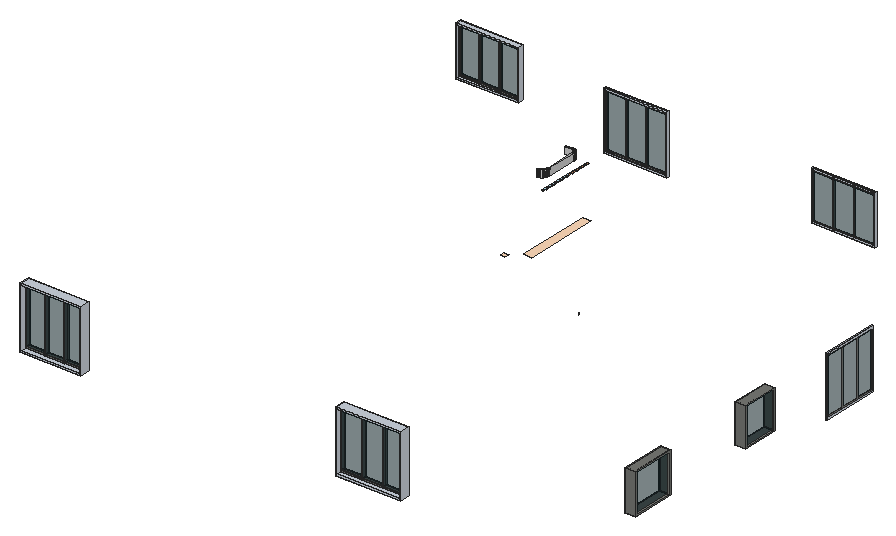
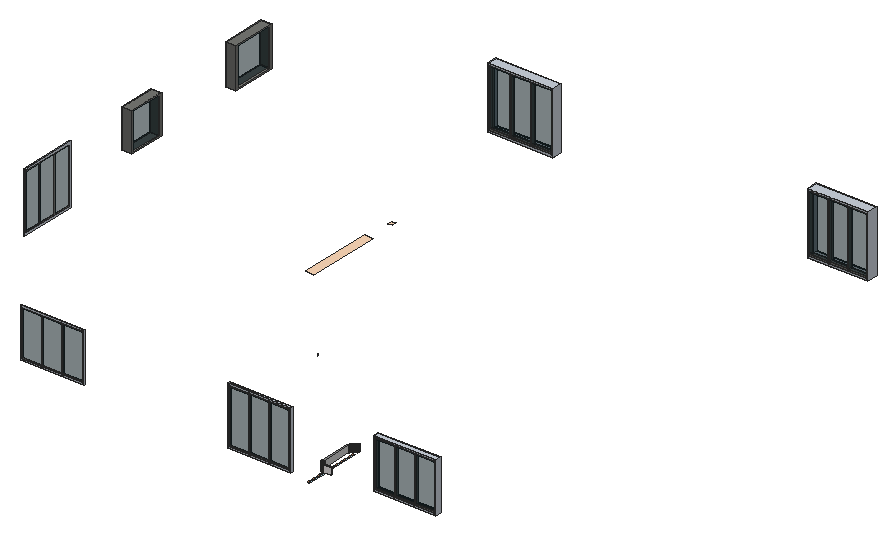
# SketchUp Ruby script. Lengths in inches.
U = 1.inch
M = Sketchup.active_model
def pt(a) = Geom::Point3d.new(a.map { |v| v * U })
def face(e, loops, mat)
  f = e.add_face(loops[0].map { |a| pt(a) })
  loops[1..].each { |l| e.add_face(l.map { |a| pt(a) }).erase! }
  f.material = f.back_material = mat if mat
  f
end
# faces: each face lists its corners as indices into pts; further lists are holes
def faces(e, pts, list, mat = nil) = list.each { |f| face(e, (f[0].is_a?(Array) ? f : [f]).map { |l| l.map { |i| pts[i] } }, mat) }
# xy, xz, yz: faces in a plane at the given z, y or x. An outline is a flat list of corners, or four numbers for a rectangle; further outlines are holes
def ring(l) = l.size == 4 ? [[l[0], l[1]], [l[2], l[1]], [l[2], l[3]], [l[0], l[3]]] : l.each_slice(2).to_a
def flat(e, list, mat, &to3) = list.each { |f| face(e, (f[0].is_a?(Array) ? f : [f]).map { |l| ring(l).map { |u, v| to3.(u, v) } }, mat) }
def xy(e, z, list, mat = nil) = flat(e, list, mat) { |x, y| [x, y, z] }
def xz(e, y, list, mat = nil) = flat(e, list, mat) { |x, z| [x, y, z] }
def yz(e, x, list, mat = nil) = flat(e, list, mat) { |y, z| [x, y, z] }
def lines(e, pts, list) = list.each { |a, b| e.add_line(pt(pts[a]), pt(pts[b])) }
# prism: a flat outline (further loops are holes) pulled along v
def prism(e, loops, v, mat = nil)
  f = face(e, loops, mat); d = Geom::Vector3d.new(v.map { |x| x * U })
  f.pushpull(f.normal.samedirection?(d) ? d.length : -d.length)
end
def box(e, o, s, mat = nil) = prism(e, [[o, [o[0] + s[0], o[1], o[2]], [o[0] + s[0], o[1] + s[1], o[2]], [o[0], o[1] + s[1], o[2]]]], [0, 0, s[2]], mat)
def at(x, y, z, deg = 0) = Geom::Transformation.translation(pt([x, y, z])) * Geom::Transformation.rotation(ORIGIN, Z_AXIS, deg.degrees)
def axes(o, x, y, z) = Geom::Transformation.new([*x, 0, *y, 0, *z, 0, *pt(o).to_a, 1])
def part(name) = M.definitions.add(name)
# library, detail: a bought-in or finely detailed component or shape, given as its bounding box
def library(name, o, s) = part(name).tap { |d| box(d.entities, o, s) }
def detail(e, o, s) = box(e.add_group.entities, o, s)
def put(e, d, t, mat = nil) = e.add_instance(d, t).tap { |i| i.material = mat if mat }
def group(e, t, mat = nil) = e.add_group.tap { |g| g.transformation = t; g.material = mat if mat }.entities
root = M.entities
M.materials.add("Material \#1").color = [140, 140, 140]
M.materials.add("[0006_Pink]").color = [255, 192, 203]
M.materials.add("[0010_Snow]").color = [255, 250, 250]
M.materials.add("[0027_PeachPuff]").color = [255, 218, 185]
M.materials.add("[0095_LightBlue]").color = [173, 216, 230]
M.materials.add("[Carrera Marble]").color = [207, 207, 207]
M.materials.add("[Metal Aluminum Anodized]").color = [202, 209, 219]
M.materials.add("[Metal Seamed]").color = [118, 119, 115]
M.materials.add("[Translucent Glass Tinted]").color = [1, 25, 30]
M.materials["[Translucent Glass Tinted]"].alpha = 0.31
M.materials.add("[Wood Veneer 02]").color = [190, 128, 91]
c1 = part("Group\#106")
prism(c1.entities,[[[0.375,0,0],[0.375,0,57],[0.375,26.94,57],[0.375,26.94,0]],[[0.375,25.82,55.875],[0.375,1.125,55.875],[0.375,1.125,1.125],[0.375,25.82,1.125]]],[1.5,0,0])
c2 = part("Group\#9")
put(c2.entities,c1,at(-0.375,0,0),"[Metal Seamed]")
g1 = group(c2.entities,at(0.18,24.32,1.125),"[Translucent Glass Tinted]")
box(g1,[0,-23.19,0],[1.125,24.69,54.75])
c3 = part("Group\#11")
box(c3.entities,[0,-23.19,0],[1.125,24.69,54.75])
c4 = part("Group\#26")
put(c4.entities,c1,at(-0.375,0,0),"[Metal Seamed]")
put(c4.entities,c3,at(0.18,24.32,1.125),"[Translucent Glass Tinted]")
c5 = part("Group\#74")
prism(c5.entities,[[[0,0,60],[0,56.89,60],[0,56.89,0],[0,0,0]],[[0,0.78,1.5],[0,56.23,1.5],[0,56.23,58.5],[0,0.78,58.5]]],[3.6875,0,0])
c6 = part("Group\#23")
put(c6.entities,c4,axes([1.875,12.09,1.5],[1,0,0],[0,1.60697,0],[0,0,1]))
put(c6.entities,c5,axes([0,-72.67,0],[1,0,0],[0,2.27742,0],[0,0,1]),"[Metal Aluminum Anodized]")
put(c6.entities,c4,axes([1.875,-70.89,1.5],[1,0,0],[0,1.60697,0],[0,0,1]))
put(c6.entities,c4,axes([1.875,-29.4,1.5],[1,0,0],[0,1.60697,0],[0,0,1]))
c7 = part("Group\#71")
g2 = group(c7.entities,at(1.875,12.09,1.5))
put(g2,c1,axes([-0.375,0,0],[1,0,0],[0,1.60697,0],[0,0,1]),"[Metal Seamed]")
put(g2,c3,axes([0.18,39.08,1.125],[1,0,0],[0,1.60697,0],[0,0,1]),"[Translucent Glass Tinted]")
put(c7.entities,c5,axes([0,-72.67,0],[1,0,0],[0,2.27742,0],[0,0,1]),"[Metal Aluminum Anodized]")
g3 = group(c7.entities,at(1.875,-70.89,1.5))
put(g3,c1,axes([-0.375,0,0],[1,0,0],[0,1.60697,0],[0,0,1]),"[Metal Seamed]")
put(g3,c3,axes([0.18,39.08,1.125],[1,0,0],[0,1.60697,0],[0,0,1]),"[Translucent Glass Tinted]")
g4 = group(c7.entities,at(1.875,-29.4,1.5))
put(g4,c1,axes([-0.375,0,0],[1,0,0],[0,1.60697,0],[0,0,1]),"[Metal Seamed]")
put(g4,c3,axes([0.18,39.08,1.125],[1,0,0],[0,1.60697,0],[0,0,1]),"[Translucent Glass Tinted]")
c8 = part("Aluminium+Channel+Glass+Window")
put(c8.entities,c2,axes([-171.39,108.96,76.09],[5.11465,0,0],[0,1.22817,0],[0,0,0.52]))
put(c8.entities,c6,axes([-283.96,456.7,67.48],[0,-0.25416,0],[0.36397,0,0],[0,0,0.60655]))
put(c8.entities,c2,axes([-171.39,211.02,76.09],[5.11465,0,0],[0,1.01722,0],[0,0,0.50603]))
g5 = group(c8.entities,at(-165.24,312.63,60.59))
put(g5,c4,axes([-0.4,3.96,1.11],[-0.21516,0,0],[0,0.5266,0],[0,0,0.73906]))
put(g5,c5,axes([0,-23.8125,0],[-0.21516,0,0],[0,0.7463,0],[0,0,0.73906]),"[Metal Aluminum Anodized]")
put(g5,c4,axes([-0.4,-23.23,1.11],[-0.21516,0,0],[0,0.5266,0],[0,0,0.73906]))
put(g5,c4,axes([-0.4,-9.63,1.11],[-0.21516,0,0],[0,0.5266,0],[0,0,0.73906]))
put(c8.entities,c6,axes([-436.19,452.97,61.625],[0,0.47782,0],[0.35744,0,0],[0,0,0.72188]))
put(c8.entities,c7,axes([-545.9,452.97,72.6875],[0,1.11491,0],[0.35744,0,0],[0,0,0.61562]))
put(c8.entities,c7,axes([-319.76,60.02,60.59],[0,2.06259,0],[0.3704,0,0],[0,0,0.76364]))
put(c8.entities,c7,axes([-555.39,59.6875,60.59],[0,2.15185,0],[0.34455,0,0],[0,0,0.76364]))
xy(root,54.75,[[263.199,488.047,263.887,509.172],[263.199,509.672,263.887,530]],"[0095_LightBlue]")
xy(root,54.75,[[263.887,488.047,264.762,489.213],[263.887,490.542,264.762,491.708],[263.887,493.037,264.762,494.203],[263.887,495.531,264.762,496.698],[263.887,498.026,264.762,499.193],
  [263.887,500.521,264.762,501.6875],[263.887,503.016,264.762,504.182],[263.887,505.511,264.762,506.677],[263.887,508.006,264.762,509.172],[263.887,510.006,264.762,511.172],
  [263.887,512.359,264.762,513.525],[263.887,514.713,264.762,515.879],[263.887,517.066,264.762,518.232],[263.887,519.42,264.762,520.586],[263.887,521.773,264.762,522.939],
  [263.887,524.127,264.762,525.293],[263.887,526.48,264.762,527.646],[263.887,528.834,264.762,530]],"[Wood Veneer 02]")
xy(root,105.529,[[358.5625,351.9375,364.5625,406.625]],"[0027_PeachPuff]")
xy(root,110.269,[[354.3125,336.471,357.4375,339.471]],"[0027_PeachPuff]")
xz(root,521.998,[[252.877,60.5,258.176,65.335]],"[Carrera Marble]")
xz(root,523.414,[[252.877,60.5,258.176,65.335]],"[0010_Snow]")
yz(root,261.26,[[496.673,60.5,518.65,65.335]],"[Carrera Marble]")
yz(root,262.563,[[496.673,60.5,518.65,65.335]],"[Carrera Marble]")
yz(root,362.669,[[398.017,47.077,397.949,47.095,397.947,47.086],[398.017,47.077,398.017,47.087,397.949,47.095],[398.017,47.077,398.087,47.086,398.017,47.087],[397.947,47.086,397.887,47.121,397.881,47.112],[397.947,47.086,397.949,47.095,397.887,47.121],
  [398.087,47.086,398.084,47.095,398.017,47.087],[398.087,47.086,398.152,47.112,398.084,47.095],[398.084,47.095,398.152,47.112,398.147,47.121],[397.881,47.112,397.833,47.161,397.825,47.154],[397.881,47.112,397.887,47.121,397.833,47.161],
  [398.152,47.112,398.208,47.154,398.147,47.121],[398.147,47.121,398.208,47.154,398.201,47.161],[397.825,47.154,397.791,47.213,397.782,47.208],[397.825,47.154,397.833,47.161,397.791,47.213],[398.208,47.154,398.251,47.208,398.201,47.161],
  [398.201,47.161,398.251,47.208,398.242,47.213],[397.782,47.208,397.765,47.275,397.755,47.272],[397.782,47.208,397.791,47.213,397.765,47.275],[398.251,47.208,398.278,47.272,398.242,47.213],[398.242,47.213,398.278,47.272,398.268,47.275],
  [397.755,47.272,397.756,47.34,397.746,47.34],[397.755,47.272,397.765,47.275,397.756,47.34],[398.278,47.272,398.288,47.34,398.268,47.275],[398.268,47.275,398.288,47.34,398.277,47.34],[397.746,47.34,397.756,47.34,397.765,47.406],
  [397.746,47.34,397.765,47.406,397.755,47.409],[398.277,47.34,398.278,47.409,398.268,47.406],[398.277,47.34,398.288,47.34,398.278,47.409],[397.765,47.406,397.791,47.467,397.755,47.409],[398.268,47.406,398.251,47.472,398.242,47.467],
  [398.268,47.406,398.278,47.409,398.251,47.472],[397.755,47.409,397.791,47.467,397.782,47.472],[397.791,47.467,397.833,47.52,397.782,47.472],[398.242,47.467,398.208,47.527,398.201,47.52],[398.242,47.467,398.251,47.472,398.208,47.527],
  [397.782,47.472,397.833,47.52,397.825,47.527],[397.833,47.52,397.887,47.56,397.825,47.527],[398.201,47.52,398.152,47.569,398.147,47.56],[398.201,47.52,398.208,47.527,398.152,47.569],[397.825,47.527,397.887,47.56,397.881,47.569],
  [397.887,47.56,397.949,47.585,397.881,47.569],[398.147,47.56,398.087,47.595,398.084,47.585],[398.147,47.56,398.152,47.569,398.087,47.595],[397.881,47.569,397.949,47.585,397.947,47.595],[397.949,47.585,398.017,47.594,397.947,47.595],
  [398.084,47.585,398.017,47.604,398.017,47.594],[398.084,47.585,398.087,47.595,398.017,47.604],[398.017,47.594,398.017,47.604,397.947,47.595]],"Material \#1")
yz(root,362.676,[[398.017,46.487,397.867,46.557,397.932,46.506],[398.017,46.487,398.167,46.557,397.867,46.557],[398.017,46.487,397.932,46.506,397.973,46.492],[398.017,46.487,398.061,46.492,398.101,46.506],[398.017,46.487,398.101,46.506,398.167,46.557],
  [397.932,46.506,397.867,46.557,397.896,46.528],[398.101,46.506,398.137,46.528,398.167,46.557],[397.867,46.557,397.824,46.675,397.829,46.632],[397.867,46.557,398.017,47.044,397.824,46.675],[397.867,46.557,397.829,46.632,397.844,46.592],
  [397.867,46.557,398.086,47.052,398.017,47.044],[397.867,46.557,398.15,47.075,398.086,47.052],[397.867,46.557,398.167,46.557,398.21,47.041],[397.867,46.557,398.207,47.109,398.15,47.075],[397.867,46.557,398.21,47.041,398.211,47.048],
  [397.867,46.557,398.211,47.048,398.213,47.055],[397.867,46.557,398.213,47.055,398.217,47.062],[397.867,46.557,398.217,47.062,398.358,47.296],[397.867,46.557,398.254,47.155,398.207,47.109],[397.867,46.557,398.358,47.296,398.254,47.155],
  [398.167,46.557,398.19,46.592,398.204,46.632],[398.167,46.557,398.204,46.632,398.209,47.033],[398.167,46.557,398.209,47.033,398.21,47.041],[398.204,46.632,398.209,46.675,398.209,47.033],[397.824,46.675,397.827,47.109,397.824,47.033],
  [397.824,46.675,397.883,47.075,397.827,47.109],[397.824,46.675,397.947,47.052,397.883,47.075],[397.824,46.675,398.017,47.044,397.947,47.052],[397.824,47.033,397.822,47.049,397.824,47.041],[397.824,47.033,397.827,47.109,397.822,47.049],
  [397.822,47.049,397.78,47.155,397.817,47.062],[397.822,47.049,397.827,47.109,397.78,47.155],[397.822,47.049,397.817,47.062,397.82,47.056],[397.817,47.062,397.676,47.296,397.812,47.068],[397.817,47.062,397.744,47.21,397.676,47.296],
  [397.817,47.062,397.78,47.155,397.744,47.21],[398.217,47.062,398.221,47.068,398.358,47.296],[397.812,47.068,397.676,47.296,397.807,47.074],[398.221,47.068,398.226,47.074,398.358,47.296],[397.807,47.074,397.676,47.296,397.742,47.141],
  [397.807,47.074,397.742,47.141,397.801,47.08],[398.226,47.074,398.233,47.08,398.293,47.14],[398.226,47.074,398.293,47.14,398.358,47.296],[397.801,47.08,397.742,47.141,397.77,47.109],[398.233,47.08,398.265,47.108,398.293,47.14],
  [398.293,47.14,398.316,47.175,398.335,47.213],[398.293,47.14,398.335,47.213,398.358,47.296],[397.742,47.141,397.676,47.296,397.699,47.214],[397.742,47.141,397.699,47.214,397.718,47.176],[398.254,47.155,398.358,47.296,398.29,47.21],
  [397.744,47.21,397.721,47.273,397.676,47.296],[398.29,47.21,398.358,47.296,398.3125,47.273],[398.335,47.213,398.349,47.253,398.358,47.296],[397.699,47.214,397.676,47.296,397.685,47.254],[397.721,47.273,397.713,47.34,397.676,47.296],
  [398.3125,47.273,398.358,47.296,398.321,47.34],[397.676,47.296,397.682,47.417,397.672,47.34],[397.676,47.296,397.713,47.34,397.721,47.408],[397.676,47.296,397.721,47.408,397.744,47.47],[397.676,47.296,397.744,47.47,397.748,47.55],
  [397.676,47.296,397.748,47.55,397.682,47.417],[398.358,47.296,398.285,47.55,398.3125,47.408],[398.358,47.296,398.352,47.417,398.285,47.55],[398.358,47.296,398.3125,47.408,398.321,47.34],[398.358,47.296,398.361,47.34,398.352,47.417],
  [398.3125,47.408,398.285,47.55,398.29,47.47],[397.682,47.417,397.748,47.55,397.707,47.488],[398.352,47.417,398.326,47.488,398.285,47.55],[397.744,47.47,397.78,47.525,397.748,47.55],[398.29,47.47,398.285,47.55,398.254,47.525],
  [397.78,47.525,397.827,47.571,397.748,47.55],[398.254,47.525,398.285,47.55,398.207,47.571],[397.748,47.55,397.827,47.571,397.883,47.606],[397.748,47.55,397.865,47.642,397.801,47.602],[397.748,47.55,397.883,47.606,398.017,47.676],
  [397.748,47.55,398.017,47.676,397.865,47.642],[398.285,47.55,398.017,47.676,398.15,47.606],[398.285,47.55,398.168,47.642,398.017,47.676],[398.285,47.55,398.15,47.606,398.207,47.571],[398.285,47.55,398.232,47.602,398.168,47.642],
  [397.883,47.606,397.947,47.628,398.017,47.676],[398.15,47.606,398.017,47.676,398.086,47.628],[397.947,47.628,398.017,47.636,398.017,47.676],[398.086,47.628,398.017,47.676,398.017,47.636],[397.865,47.642,398.017,47.676,397.938,47.667],
  [398.168,47.642,398.096,47.667,398.017,47.676]],"Material \#1")
p = [[257.338,491.001,60.5],[258.02,491.049,60.5],[258.02,491.049,65.335],[257.338,491.001,65.335],[258.691,491.194,60.5],[258.691,491.194,65.335],
  [259.338,491.432,60.5],[259.338,491.432,65.335],[259.951,491.761,60.5],[259.951,491.761,65.335],[260.519,492.173,60.5],[260.519,492.173,65.335],
  [261.033,492.662,60.5],[261.033,492.662,65.335],[257.85,492.452,60.5],[257.338,492.416,60.5],[257.338,492.416,65.335],[257.85,492.452,65.335],
  [258.353,492.561,60.5],[258.353,492.561,65.335],[258.839,492.74,60.5],[258.839,492.74,65.335],[259.299,492.986,60.5],[259.299,492.986,65.335],
  [261.484,493.22,60.5],[261.484,493.22,65.335],[259.726,493.296,60.5],[259.726,493.296,65.335],[261.863,493.837,60.5],[261.863,493.837,65.335],
  [260.111,493.663,60.5],[260.111,493.663,65.335],[260.449,494.082,60.5],[260.449,494.082,65.335],[262.166,494.503,60.5],[262.166,494.503,65.335],
  [260.734,494.545,60.5],[260.734,494.545,65.335],[260.961,495.044,60.5],[260.961,495.044,65.335],[262.385,495.205,60.5],[262.385,495.205,65.335],
  [261.126,495.572,60.5],[261.126,495.572,65.335],[262.519,495.933,60.5],[262.519,495.933,65.335],[261.226,496.118,60.5],[261.226,496.118,65.335],
  [262.563,496.673,60.5],[262.563,496.673,65.335],[261.26,496.673,60.5],[261.26,496.673,65.335],[261.233,519.087,60.5],[261.26,518.65,60.5],
  [261.26,518.65,65.335],[261.233,519.087,65.335],[262.563,518.65,60.5],[262.526,519.272,60.5],[262.526,519.272,65.335],[262.563,518.65,65.335],
  [261.155,519.517,60.5],[261.155,519.517,65.335],[262.414,519.883,60.5],[262.414,519.883,65.335],[261.025,519.931,60.5],[261.025,519.931,65.335],
  [260.847,520.324,60.5],[260.847,520.324,65.335],[262.23,520.473,60.5],[262.23,520.473,65.335],[260.623,520.688,60.5],[260.623,520.688,65.335],
  [261.976,521.032,60.5],[261.976,521.032,65.335],[260.357,521.018,60.5],[260.357,521.018,65.335],[260.053,521.306,60.5],[260.053,521.306,65.335],
  [261.657,521.55,60.5],[261.657,521.55,65.335],[259.718,521.55,60.5],[259.718,521.55,65.335],[259.356,521.743,60.5],[259.356,521.743,65.335],
  [261.278,522.018,60.5],[261.278,522.018,65.335],[258.974,521.884,60.5],[258.974,521.884,65.335],[258.579,521.969,60.5],[258.579,521.969,65.335],
  [258.176,521.998,60.5],[258.176,521.998,65.335],[260.847,522.429,60.5],[260.847,522.429,65.335],[260.37,522.775,60.5],[260.37,522.775,65.335],
  [259.855,523.051,60.5],[259.855,523.051,65.335],[259.312,523.251,60.5],[259.312,523.251,65.335],[258.749,523.373,60.5],[258.749,523.373,65.335],
  [258.176,523.414,60.5],[258.176,523.414,65.335]]
faces(root,p,[[0,1,2,3],[1,4,5,2],[4,6,7,5],[6,8,9,7],[8,10,11,9],[10,12,13,11],[14,15,16,17],[18,14,17,19],
  [20,18,19,21],[22,20,21,23],[12,24,25,13],[26,22,23,27],[24,28,29,25],[30,26,27,31],[32,30,31,33],[28,34,35,29],
  [36,32,33,37],[38,36,37,39],[34,40,41,35],[42,38,39,43],[40,44,45,41],[46,42,43,47],[44,48,49,45],[50,46,47,51],
  [52,53,54,55],[56,57,58,59],[60,52,55,61],[57,62,63,58],[64,60,61,65],[66,64,65,67],[62,68,69,63],[70,66,67,71],
  [68,72,73,69],[74,70,71,75],[76,74,75,77],[72,78,79,73],[80,76,77,81],[82,80,81,83],[78,84,85,79],[86,82,83,87],
  [88,86,87,89],[90,88,89,91],[84,92,93,85],[92,94,95,93],[94,96,97,95],[96,98,99,97],[98,100,101,99],[100,102,103,101]],"[Carrera Marble]")
put(root,c8,at(733.82,82.34,0),"[0006_Pink]")
